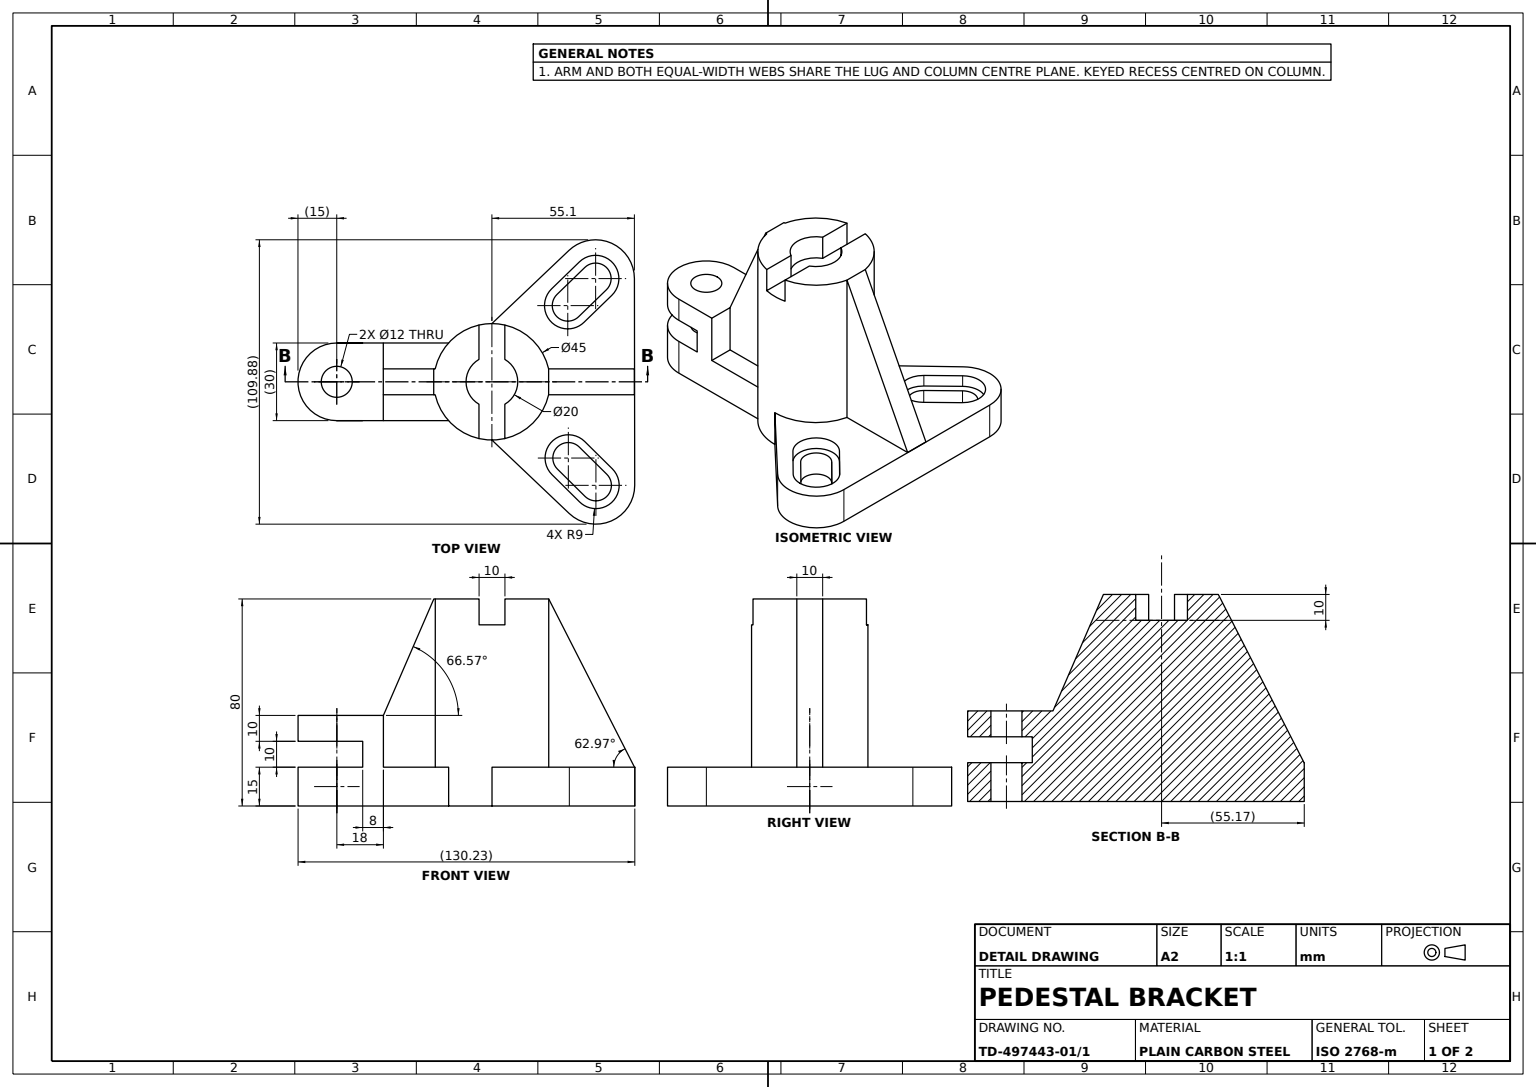
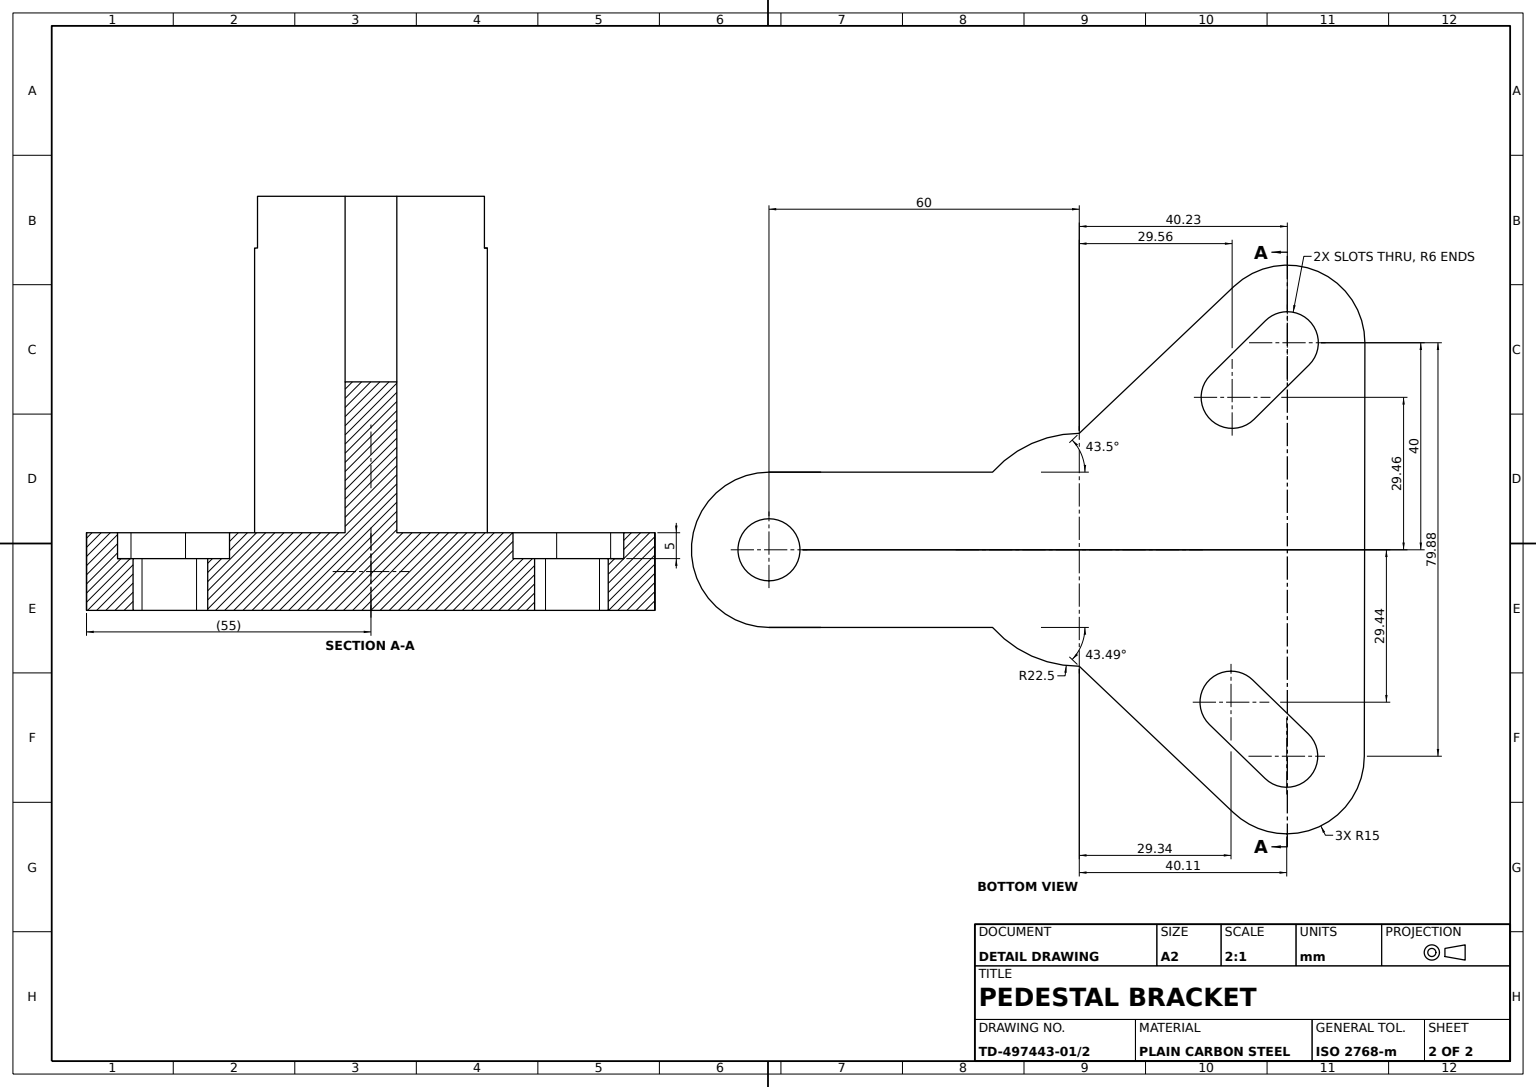
solid
v1 (-5,70,21.937411)
v2 (5,70,21.937411)
e1 v1 v2 CIRCLE(AX(P(0,70,0),D(0,1,0),D(0,0,1)),22.5)
v3 (-5,80,21.937411)
e2 v1 v3 LINE
v4 (-21.937411,80,5)
e3 v4 v3 CIRCLE(AX(P(0,80,0),D(0,1,0),D(0,0,1)),22.5)
v5 (-21.937411,15,5)
e4 v4 v5 LINE
v6 (-16.77051,15,15)
e5 v5 v6 CIRCLE(AX(P(0,15,0),D(0,1,0),D(0,0,1)),22.5)
v7 (-16.77051,0,15)
e6 v6 v7 LINE
v8 (0,0,22.5)
e7 v7 v8 CIRCLE(AX(P(0,0,0),D(0,1,0),D(0,0,1)),22.5)
v9 (0,15,22.5)
e8 v9 v8 LINE
v10 (21.937411,15,5)
e9 v10 v9 CIRCLE(AX(P(0,15,0),D(0,-1,0),D(0,0,1)),22.5)
v11 (21.937411,80,5)
e10 v11 v10 LINE
v12 (5,80,21.937411)
e11 v12 v11 CIRCLE(AX(P(0,80,0),D(0,1,0),D(0,0,1)),22.5)
e12 v12 v2 LINE
face CYL(AX(P(0,80,0),D(0,-1,0),D(0,0,-1)),22.5) [-e1 e2 -e3 e4 e5 e6 e7 -e8 -e9 -e10 -e11 e12]
v13 (55.113655,15,-39.880202)
v14 (55.113655,0,-39.880202)
e13 v13 v14 LINE
v15 (40.113655,0,-54.880202)
e14 v14 v15 CIRCLE(AX(P(40.113655,0,-39.880202),D(0,1,0),D(0,0,1)),15)
v16 (40.113655,15,-54.880202)
e15 v16 v15 LINE
e16 v13 v16 CIRCLE(AX(P(40.113655,15,-39.880202),D(0,1,0),D(0,0,1)),15)
face CYL(AX(P(40.113655,15,-39.880202),D(0,-1,0),D(0,0,-1)),15) [e13 e14 -e15 -e16]
v17 (29.901541,0,50.879576)
e17 v8 v17 LINE
v18 (29.901541,15,50.879576)
e18 v18 v17 LINE
e19 v9 v18 LINE
face PLANE(AX(P(-11.234667,15,11.837169),D(0.688406563,0,-0.725325034),D(-0.725325034,0,-0.688406563))) rev [e8 e17 -e18 -e19]
v19 (29.340903,10,-20.442395)
v20 (35.603587,10,-22.978744)
e20 v19 v20 CIRCLE(AX(P(29.340903,10,-29.442395),D(0,1,0),D(0,0,1)),9)
v21 (29.340903,15,-20.442395)
e21 v19 v21 LINE
v22 (35.603587,15,-22.978744)
e22 v21 v22 CIRCLE(AX(P(29.340903,15,-29.442395),D(0,1,0),D(0,0,1)),9)
e23 v20 v22 LINE
face CYL(AX(P(29.340903,10,-29.442395),D(0,1,0),D(0,0,1)),9) rev [-e20 e21 e22 -e23]
v23 (55.1,15,5)
e24 v23 v11 LINE
e25 v23 v10 LINE
face PLANE(AX(P(55.1,80,5),D(0,0,-1),D(-1,0,0))) rev [e24 e10 -e25]
v24 (21.937411,80,-5)
v25 (5,80,-21.937411)
e26 v24 v25 CIRCLE(AX(P(0,80,0),D(0,1,0),D(0,0,1)),22.5)
v26 (21.937411,15,-5)
e27 v26 v24 LINE
v27 (0,15,-22.5)
e28 v27 v26 CIRCLE(AX(P(0,15,0),D(0,-1,0),D(0,0,1)),22.5)
v28 (0,70,-22.5)
e29 v28 v27 LINE
v29 (5,70,-21.937411)
e30 v29 v28 CIRCLE(AX(P(0,70,0),D(0,1,0),D(0,0,1)),22.5)
e31 v29 v25 LINE
face CYL(AX(P(0,80,0),D(0,-1,0),D(0,0,-1)),22.5) [-e26 -e27 -e28 -e29 -e30 e31]
v30 (44.444996,0,35.731925)
v31 (44.444996,10,35.731925)
e32 v30 v31 LINE
v32 (40.227639,0,45.999701)
e33 v32 v30 CIRCLE(AX(P(40.227639,0,39.999701),D(0,1,0),D(0,0,1)),6)
v33 (40.227639,10,45.999701)
e34 v32 v33 LINE
e35 v33 v31 CIRCLE(AX(P(40.227639,10,39.999701),D(0,1,0),D(0,0,1)),6)
face CYL(AX(P(40.227639,0,39.999701),D(0,1,0),D(0,0,1)),6) rev [-e32 -e33 e34 e35]
v34 (-5,80,8.660254)
e36 v34 v3 LINE
v35 (-5,80,-8.660254)
e37 v35 v34 CIRCLE(AX(P(0,80,0),D(0,1,0),D(0,0,1)),10)
v36 (-5,80,-21.937411)
e38 v36 v35 LINE
v37 (-21.937411,80,-5)
e39 v36 v37 CIRCLE(AX(P(0,80,0),D(0,1,0),D(0,0,1)),22.5)
v38 (-22.5,80,-5)
e40 v37 v38 LINE
v39 (-22.5,80,5)
e41 v38 v39 LINE
e42 v4 v39 LINE
face PLANE(AX(P(0,80,0),D(0,1,0),D(0,0,1))) [-e36 -e37 -e38 e39 e40 e41 -e42 e3]
v40 (-60,15,15)
v41 (-50,15,15)
e43 v40 v41 LINE
v42 (-50,15,-15)
e44 v42 v41 LINE
v43 (-60,15,-15)
e45 v42 v43 LINE
e46 v43 v40 CIRCLE(AX(P(-60,15,0),D(0,1,0),D(0,0,1)),15)
v44 (-60,15,6)
v45 (-60,15,-6)
e47 v44 v45 CIRCLE(AX(P(-60,15,0),D(0,1,0),D(0,0,1)),6)
e48 v45 v44 CIRCLE(AX(P(-60,15,0),D(0,1,0),D(0,0,1)),6)
face PLANE(AX(P(-60,15,0),D(0,1,0),D(0,0,1))) [e43 -e44 e45 e46] [-e47 -e48]
v46 (-42,15,5)
v47 (-42,15,15)
e49 v46 v47 LINE
e50 v47 v6 LINE
e51 v46 v5 LINE
face PLANE(AX(P(-60,15,0),D(0,1,0),D(0,0,1))) [e49 e50 -e5 -e51]
v48 (-21.937411,15,-5)
e52 v37 v48 LINE
v49 (-42,15,-5)
e53 v49 v48 LINE
v50 (-42,35,-5)
e54 v50 v49 LINE
e55 v38 v50 LINE
face PLANE(AX(P(-9.88618,40,-5),D(0,0,1),D(1,0,0))) rev [-e40 e52 -e53 -e54 -e55]
v51 (25.16578,0,-33.751496)
v52 (25.16578,10,-33.751496)
e56 v51 v52 LINE
v53 (35.938532,0,-44.189303)
e57 v53 v51 LINE
v54 (35.938532,10,-44.189303)
e58 v53 v54 LINE
e59 v54 v52 LINE
face PLANE(AX(P(35.938532,0,-44.189303),D(-0.695853804,0,-0.718183461),D(-0.718183461,0,0.695853804))) rev [-e56 -e57 e58 e59]
v55 (-5,70,8.660254)
e60 v55 v34 LINE
e61 v55 v1 LINE
face PLANE(AX(P(-5,70,24),D(-1,0,0),D(0,0,1))) rev [e60 e36 -e2 -e61]
v56 (-60,0,-6)
e62 v56 v45 LINE
v57 (-60,0,6)
e63 v57 v56 CIRCLE(AX(P(-60,0,0),D(0,1,0),D(0,0,1)),6)
e64 v57 v44 LINE
face CYL(AX(P(-60,0,0),D(0,1,0),D(0,0,1)),6) rev [-e62 -e63 e64 e47]
v58 (33.775557,0,25.188535)
e65 v30 v58 LINE
v59 (33.775557,10,25.188535)
e66 v31 v59 LINE
e67 v58 v59 LINE
face PLANE(AX(P(44.444996,0,35.731925),D(0.702892707,0,-0.71129589),D(-0.71129589,0,-0.702892707))) rev [-e65 e32 e66 -e67]
e68 v56 v57 CIRCLE(AX(P(-60,0,0),D(0,1,0),D(0,0,1)),6)
face CYL(AX(P(-60,0,0),D(0,1,0),D(0,0,1)),6) rev [e62 e48 -e64 -e68]
v60 (-60,25,-6)
v61 (-60,25,6)
e69 v60 v61 CIRCLE(AX(P(-60,25,0),D(0,1,0),D(0,0,1)),6)
e70 v61 v60 CIRCLE(AX(P(-60,25,0),D(0,1,0),D(0,0,1)),6)
v62 (-60,25,-15)
v63 (-60,25,15)
e71 v62 v63 CIRCLE(AX(P(-60,25,0),D(0,1,0),D(0,0,1)),15)
v64 (-50,25,-15)
e72 v64 v62 LINE
v65 (-50,25,15)
e73 v64 v65 LINE
e74 v63 v65 LINE
face PLANE(AX(P(-60,25,0),D(0,1,0),D(0,0,1))) rev [e69 e70] [-e71 -e72 e73 -e74]
e75 v64 v42 LINE
v66 (-60,35,-15)
e76 v66 v62 LINE
v67 (-42,35,-15)
e77 v67 v66 LINE
v68 (-42,15,-15)
e78 v67 v68 LINE
v69 (-16.77051,15,-15)
e79 v69 v68 LINE
v70 (-16.77051,0,-15)
e80 v69 v70 LINE
v71 (-60,0,-15)
e81 v70 v71 LINE
e82 v43 v71 LINE
face PLANE(AX(P(-60,15,-15),D(0,0,1),D(1,0,0))) rev [-e75 e72 -e76 -e77 e78 -e79 e80 e81 -e82 -e45]
v72 (-60,0,15)
e83 v71 v72 CIRCLE(AX(P(-60,0,0),D(0,1,0),D(0,0,1)),15)
e84 v40 v72 LINE
face CYL(AX(P(-60,15,0),D(0,-1,0),D(0,0,-1)),15) [e83 -e84 -e46 e82]
v73 (55.1,15,-5)
e85 v73 v26 LINE
e86 v73 v24 LINE
face PLANE(AX(P(55.1,80,-5),D(0,0,1),D(0,-1,0))) rev [e85 e27 -e86]
v74 (-5,70,-21.937411)
v75 (-5,70,-8.660254)
e87 v74 v75 LINE
e88 v75 v55 CIRCLE(AX(P(0,70,0),D(0,1,0),D(0,0,1)),10)
v76 (5,70,8.660254)
e89 v2 v76 LINE
v77 (5,70,-8.660254)
e90 v76 v77 CIRCLE(AX(P(0,70,0),D(0,1,0),D(0,0,1)),10)
e91 v77 v29 LINE
e92 v28 v74 CIRCLE(AX(P(0,70,0),D(0,1,0),D(0,0,1)),22.5)
face PLANE(AX(P(0,70,0),D(0,1,0),D(0,0,1))) [e87 e88 e61 e1 e89 e90 e91 e30 e92]
v78 (0,0,-22.5)
e93 v78 v70 CIRCLE(AX(P(0,0,0),D(0,1,0),D(0,0,1)),22.5)
e94 v69 v48 CIRCLE(AX(P(0,15,0),D(0,1,0),D(0,0,1)),22.5)
e95 v36 v74 LINE
e96 v27 v78 LINE
face CYL(AX(P(0,80,0),D(0,-1,0),D(0,0,-1)),22.5) [e93 -e80 e94 -e52 -e39 e95 -e92 e29 e96]
v79 (23.232167,10,35.857973)
v80 (23.232167,15,35.857973)
e97 v79 v80 LINE
v81 (35.884235,10,23.054647)
e98 v81 v79 CIRCLE(AX(P(29.558201,10,29.45631),D(0,1,0),D(0,0,1)),9)
v82 (35.884235,15,23.054647)
e99 v81 v82 LINE
e100 v82 v80 CIRCLE(AX(P(29.558201,15,29.45631),D(0,1,0),D(0,0,1)),9)
face CYL(AX(P(29.558201,10,29.45631),D(0,1,0),D(0,0,1)),9) rev [-e97 -e98 e99 e100]
e101 v11 v24 LINE
e102 v23 v73 LINE
face PLANE(AX(P(21.937411,80,29.1),D(-0.890765621,-0.454462988,0),D(0.454462988,-0.890765621,0))) rev [e86 -e101 -e24 e102]
v83 (-60,35,6)
e103 v61 v83 LINE
v84 (-60,35,-6)
e104 v60 v84 LINE
e105 v84 v83 CIRCLE(AX(P(-60,35,0),D(0,1,0),D(0,0,1)),6)
face CYL(AX(P(-60,25,0),D(0,1,0),D(0,0,1)),6) rev [-e103 -e69 e104 e105]
v85 (33.850971,10,-46.343853)
v86 (23.078219,10,-35.906046)
e106 v85 v86 LINE
v87 (33.850971,15,-46.343853)
e107 v85 v87 LINE
v88 (23.078219,15,-35.906046)
e108 v87 v88 LINE
e109 v86 v88 LINE
face PLANE(AX(P(33.850971,10,-46.343853),D(-0.695853804,0,-0.718183461),D(-0.718183461,0,0.695853804))) rev [-e106 e107 e108 -e109]
e110 v68 v49 LINE
face PLANE(AX(P(-60,15,0),D(0,1,0),D(0,0,1))) [-e94 e79 e110 e53]
v89 (-42,35,5)
e111 v89 v46 LINE
e112 v39 v89 LINE
face PLANE(AX(P(-9.88618,40,5),D(0,0,1),D(1,0,0))) [e111 e51 -e4 e42 e112]
v90 (5,80,-8.660254)
e113 v77 v90 LINE
e114 v90 v25 LINE
face PLANE(AX(P(5,70,-8.660254),D(1,0,0),D(0,0,-1))) rev [-e31 -e91 e113 e114]
e115 v75 v35 LINE
face CYL(AX(P(0,70,0),D(0,1,0),D(0,0,1)),10) rev [-e60 -e88 e115 e37]
v91 (33.901605,15,46.401364)
e116 v80 v91 LINE
v92 (33.901605,10,46.401364)
e117 v92 v91 LINE
e118 v79 v92 LINE
face PLANE(AX(P(33.901605,10,46.401364),D(-0.702892707,0,0.71129589),D(0.71129589,0,0.702892707))) rev [e116 -e117 -e118 e97]
v93 (40.227639,15,48.999701)
e119 v91 v93 CIRCLE(AX(P(40.227639,15,39.999701),D(0,1,0),D(0,0,1)),9)
v94 (40.227639,10,48.999701)
e120 v94 v93 LINE
e121 v92 v94 CIRCLE(AX(P(40.227639,10,39.999701),D(0,1,0),D(0,0,1)),9)
face CYL(AX(P(40.227639,10,39.999701),D(0,1,0),D(0,0,1)),9) rev [e117 e119 -e120 -e121]
v95 (29.340903,0,-23.442395)
v96 (29.340903,10,-23.442395)
e122 v95 v96 LINE
v97 (33.516026,10,-25.133294)
e123 v96 v97 CIRCLE(AX(P(29.340903,10,-29.442395),D(0,1,0),D(0,0,1)),6)
v98 (33.516026,0,-25.133294)
e124 v98 v97 LINE
e125 v95 v98 CIRCLE(AX(P(29.340903,0,-29.442395),D(0,1,0),D(0,0,1)),6)
face CYL(AX(P(29.340903,0,-29.442395),D(0,1,0),D(0,0,1)),6) rev [e122 e123 -e124 -e125]
v99 (44.288778,10,-35.571101)
e126 v97 v99 LINE
v100 (44.288778,0,-35.571101)
e127 v100 v99 LINE
e128 v98 v100 LINE
face PLANE(AX(P(44.288778,0,-35.571101),D(0.695853804,0,0.718183461),D(0.718183461,0,-0.695853804))) rev [e126 -e127 -e128 e124]
e129 v50 v67 LINE
face PLANE(AX(P(-42,25,0),D(1,0,0),D(0,0,-1))) [-e129 e54 -e110 -e78]
v101 (46.376339,10,-33.416551)
e130 v20 v101 LINE
e131 v101 v85 CIRCLE(AX(P(40.113655,10,-39.880202),D(0,1,0),D(0,0,1)),9)
e132 v86 v19 CIRCLE(AX(P(29.340903,10,-29.442395),D(0,1,0),D(0,0,1)),9)
e133 v99 v54 CIRCLE(AX(P(40.113655,10,-39.880202),D(0,1,0),D(0,0,1)),6)
e134 v52 v96 CIRCLE(AX(P(29.340903,10,-29.442395),D(0,1,0),D(0,0,1)),6)
face PLANE(AX(P(40.113655,10,-39.880202),D(0,1,0),D(0,0,1))) [e130 e131 e106 e132 e20] [-e133 -e126 -e123 -e134 -e59]
v102 (55.227624,15,39.978294)
v103 (55.227624,0,39.978294)
e135 v102 v103 LINE
e136 v18 v102 CIRCLE(AX(P(40.227639,15,39.999701),D(0,1,0),D(0,0,1)),15)
e137 v17 v103 CIRCLE(AX(P(40.227639,0,39.999701),D(0,1,0),D(0,0,1)),15)
face CYL(AX(P(40.227639,15,39.999701),D(0,-1,0),D(0,0,-1)),15) [-e135 -e136 e18 e137]
v104 (36.010283,0,44.267476)
e138 v104 v32 CIRCLE(AX(P(40.227639,0,39.999701),D(0,1,0),D(0,0,1)),6)
v105 (36.010283,10,44.267476)
e139 v104 v105 LINE
e140 v105 v33 CIRCLE(AX(P(40.227639,10,39.999701),D(0,1,0),D(0,0,1)),6)
face CYL(AX(P(40.227639,0,39.999701),D(0,1,0),D(0,0,1)),6) rev [-e138 e139 e140 -e34]
v106 (5,80,8.660254)
e141 v12 v106 LINE
e142 v76 v106 LINE
face PLANE(AX(P(5,70,24),D(1,0,0),D(0,0,-1))) rev [-e12 e141 -e142 -e89]
face PLANE(AX(P(-5,70,-8.660254),D(-1,0,0),D(0,0,1))) rev [e38 -e115 -e87 -e95]
e143 v51 v95 CIRCLE(AX(P(29.340903,0,-29.442395),D(0,1,0),D(0,0,1)),6)
e144 v100 v53 CIRCLE(AX(P(40.113655,0,-39.880202),D(0,1,0),D(0,0,1)),6)
v107 (25.340845,0,33.724085)
e145 v58 v107 CIRCLE(AX(P(29.558201,0,29.45631),D(0,1,0),D(0,0,1)),6)
e146 v107 v104 LINE
e147 v72 v7 LINE
v108 (29.789731,0,-50.762141)
e148 v78 v108 LINE
e149 v15 v108 CIRCLE(AX(P(40.113655,0,-39.880202),D(0,1,0),D(0,0,1)),15)
e150 v14 v103 LINE
face PLANE(AX(P(0,0,0),D(0,1,0),D(0,0,1))) rev [e57 e143 e125 e128 e144] [e65 e145 e146 e138 e33] [e63 e68] [-e7 -e147 -e83 -e81 -e93 e148 -e149 -e14 e150 -e137 -e17]
v109 (-42,35,15)
e151 v109 v47 LINE
v110 (-60,35,15)
e152 v110 v109 LINE
e153 v110 v63 LINE
e154 v65 v41 LINE
face PLANE(AX(P(-16.77051,15,15),D(0,0,-1),D(-1,0,0))) rev [-e43 e84 e147 -e6 -e50 -e151 -e152 e153 e74 e154]
e155 v109 v89 LINE
face PLANE(AX(P(-42,25,0),D(1,0,0),D(0,0,-1))) [-e49 -e111 -e155 e151]
v111 (46.553674,10,33.598038)
v112 (46.553674,15,33.598038)
e156 v111 v112 LINE
e157 v94 v111 CIRCLE(AX(P(40.227639,10,39.999701),D(0,1,0),D(0,0,1)),9)
e158 v93 v112 CIRCLE(AX(P(40.227639,15,39.999701),D(0,1,0),D(0,0,1)),9)
face CYL(AX(P(40.227639,10,39.999701),D(0,1,0),D(0,0,1)),9) rev [-e156 -e157 e120 e158]
v113 (46.376339,15,-33.416551)
e159 v101 v113 LINE
e160 v113 v87 CIRCLE(AX(P(40.113655,15,-39.880202),D(0,1,0),D(0,0,1)),9)
face CYL(AX(P(40.113655,10,-39.880202),D(0,1,0),D(0,0,1)),9) rev [e159 e160 -e107 -e131]
e161 v66 v110 CIRCLE(AX(P(-60,35,0),D(0,1,0),D(0,0,1)),15)
face CYL(AX(P(-60,35,0),D(0,-1,0),D(0,0,-1)),15) [-e153 -e161 e76 e71]
face PLANE(AX(P(-50,25,0),D(1,0,0),D(0,0,-1))) rev [-e73 e75 e44 -e154]
e162 v106 v90 CIRCLE(AX(P(0,80,0),D(0,1,0),D(0,0,1)),10)
face PLANE(AX(P(0,80,0),D(0,1,0),D(0,0,1))) [-e141 e11 e101 e26 -e114 -e162]
e163 v112 v82 LINE
e164 v111 v81 LINE
face PLANE(AX(P(46.553674,10,33.598038),D(0.702892707,0,-0.71129589),D(-0.71129589,0,-0.702892707))) rev [e156 e163 -e99 -e164]
e165 v83 v84 CIRCLE(AX(P(-60,35,0),D(0,1,0),D(0,0,1)),6)
face CYL(AX(P(-60,25,0),D(0,1,0),D(0,0,1)),6) rev [-e70 e103 e165 -e104]
v114 (29.789731,15,-50.762141)
e166 v16 v114 CIRCLE(AX(P(40.113655,15,-39.880202),D(0,1,0),D(0,0,1)),15)
e167 v114 v108 LINE
face CYL(AX(P(40.113655,15,-39.880202),D(0,-1,0),D(0,0,-1)),15) [-e166 e15 e149 -e167]
face CYL(AX(P(0,70,0),D(0,1,0),D(0,0,1)),10) rev [e142 e162 -e113 -e90]
e168 v27 v114 LINE
e169 v13 v102 LINE
e170 v22 v113 LINE
e171 v88 v21 CIRCLE(AX(P(29.340903,15,-29.442395),D(0,1,0),D(0,0,1)),9)
face PLANE(AX(P(0,15,0),D(0,1,0),D(0,0,1))) [e166 -e168 e28 -e85 -e102 e25 e9 e19 e136 -e169 e16] [-e158 -e119 -e116 -e100 -e163] [-e160 -e170 -e22 -e171 -e108]
face CYL(AX(P(29.340903,0,-29.442395),D(0,1,0),D(0,0,1)),6) rev [e56 e134 -e122 -e143]
v115 (25.340845,10,33.724085)
e172 v59 v115 CIRCLE(AX(P(29.558201,10,29.45631),D(0,1,0),D(0,0,1)),6)
e173 v107 v115 LINE
face CYL(AX(P(29.558201,0,29.45631),D(0,1,0),D(0,0,1)),6) rev [e67 e172 -e173 -e145]
face CYL(AX(P(29.340903,10,-29.442395),D(0,1,0),D(0,0,1)),9) rev [-e132 e109 e171 -e21]
face PLANE(AX(P(-11.234431,15,-11.84166),D(-0.688261564,0,-0.725462624),D(-0.725462624,0,0.688261564))) [e168 e167 -e148 -e96]
face PLANE(AX(P(55.170457,15,-0.078736),D(0.999998982,0,-0.001427138),D(-0.001427138,0,-0.999998982))) [-e150 -e13 e169 e135]
face PLANE(AX(P(46.376339,10,-33.416551),D(0.695853804,0,0.718183461),D(0.718183461,0,-0.695853804))) rev [-e159 -e130 e23 e170]
e174 v115 v105 LINE
face PLANE(AX(P(40.227639,10,39.999701),D(0,1,0),D(0,0,1))) [-e174 -e172 -e66 -e35 -e140] [e121 e157 e164 e98 e118]
face PLANE(AX(P(36.010283,0,44.267476),D(-0.702892707,0,0.71129589),D(0.71129589,0,0.702892707))) rev [-e139 -e146 e173 e174]
e175 v89 v50 LINE
face PLANE(AX(P(-60,35,0),D(0,1,0),D(0,0,1))) [-e105 -e165] [e77 e161 e152 e155 e175 e129]
face CYL(AX(P(40.113655,0,-39.880202),D(0,1,0),D(0,0,1)),6) rev [-e58 -e144 e127 e133]
face PLANE(AX(P(-22.5,80,0),D(-0.917555625,0.397607438,0),D(-0.397607438,-0.917555625,0))) [-e41 e55 -e175 -e112]
